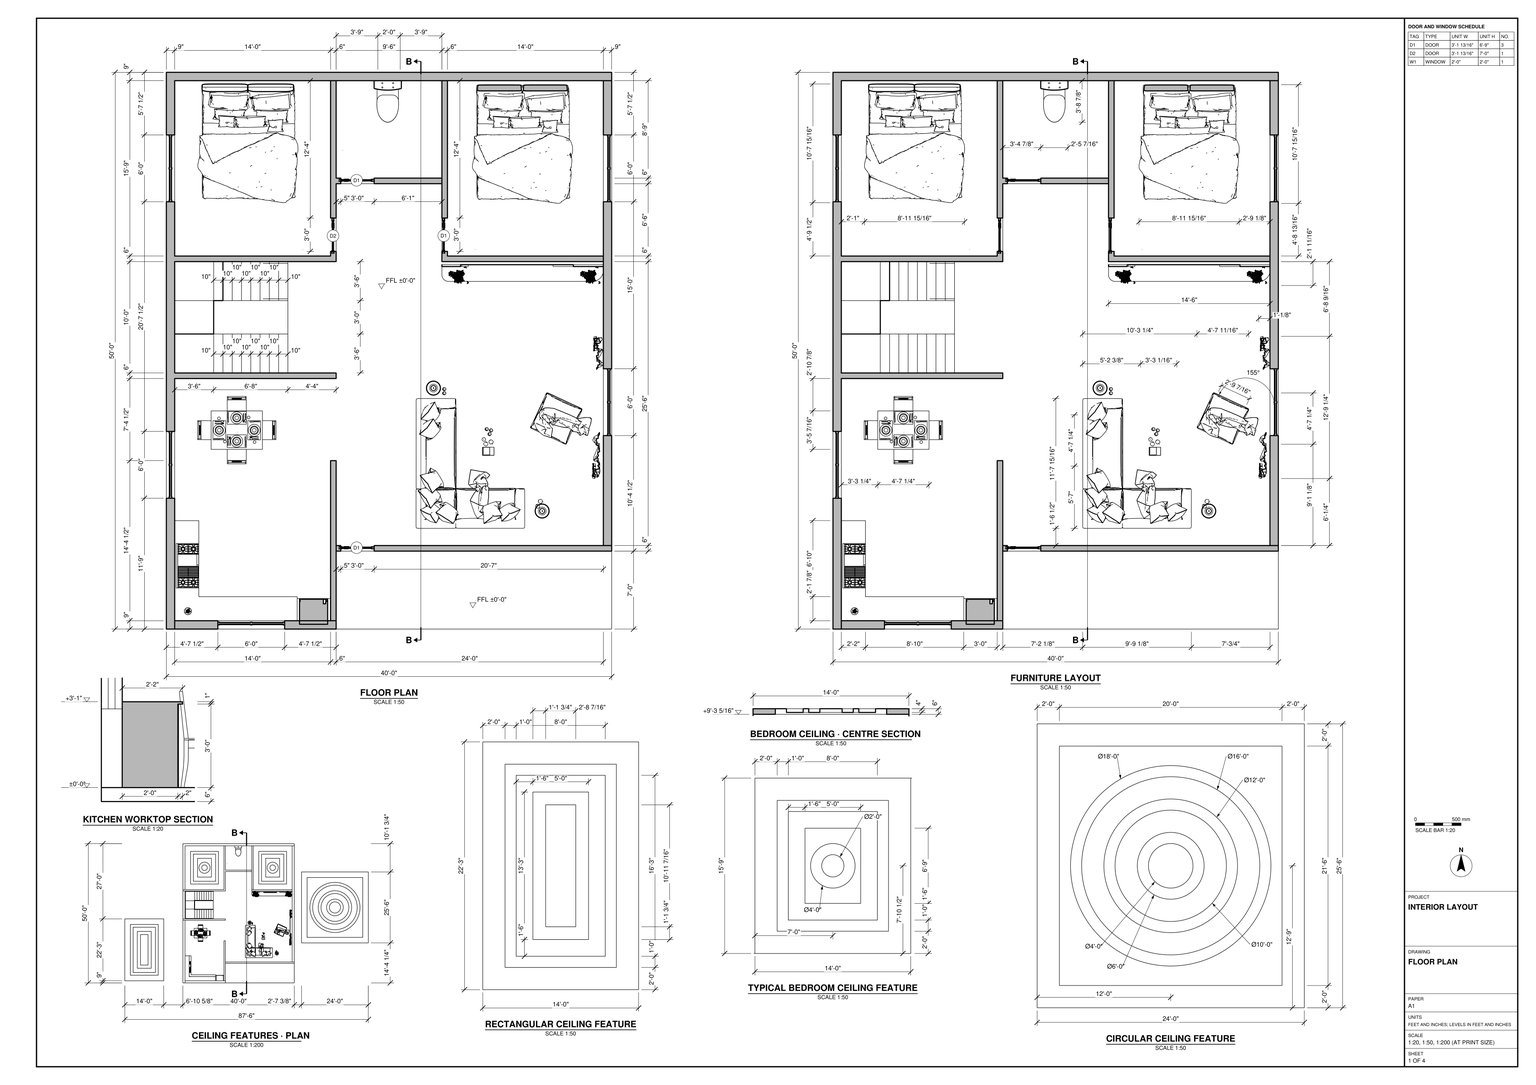
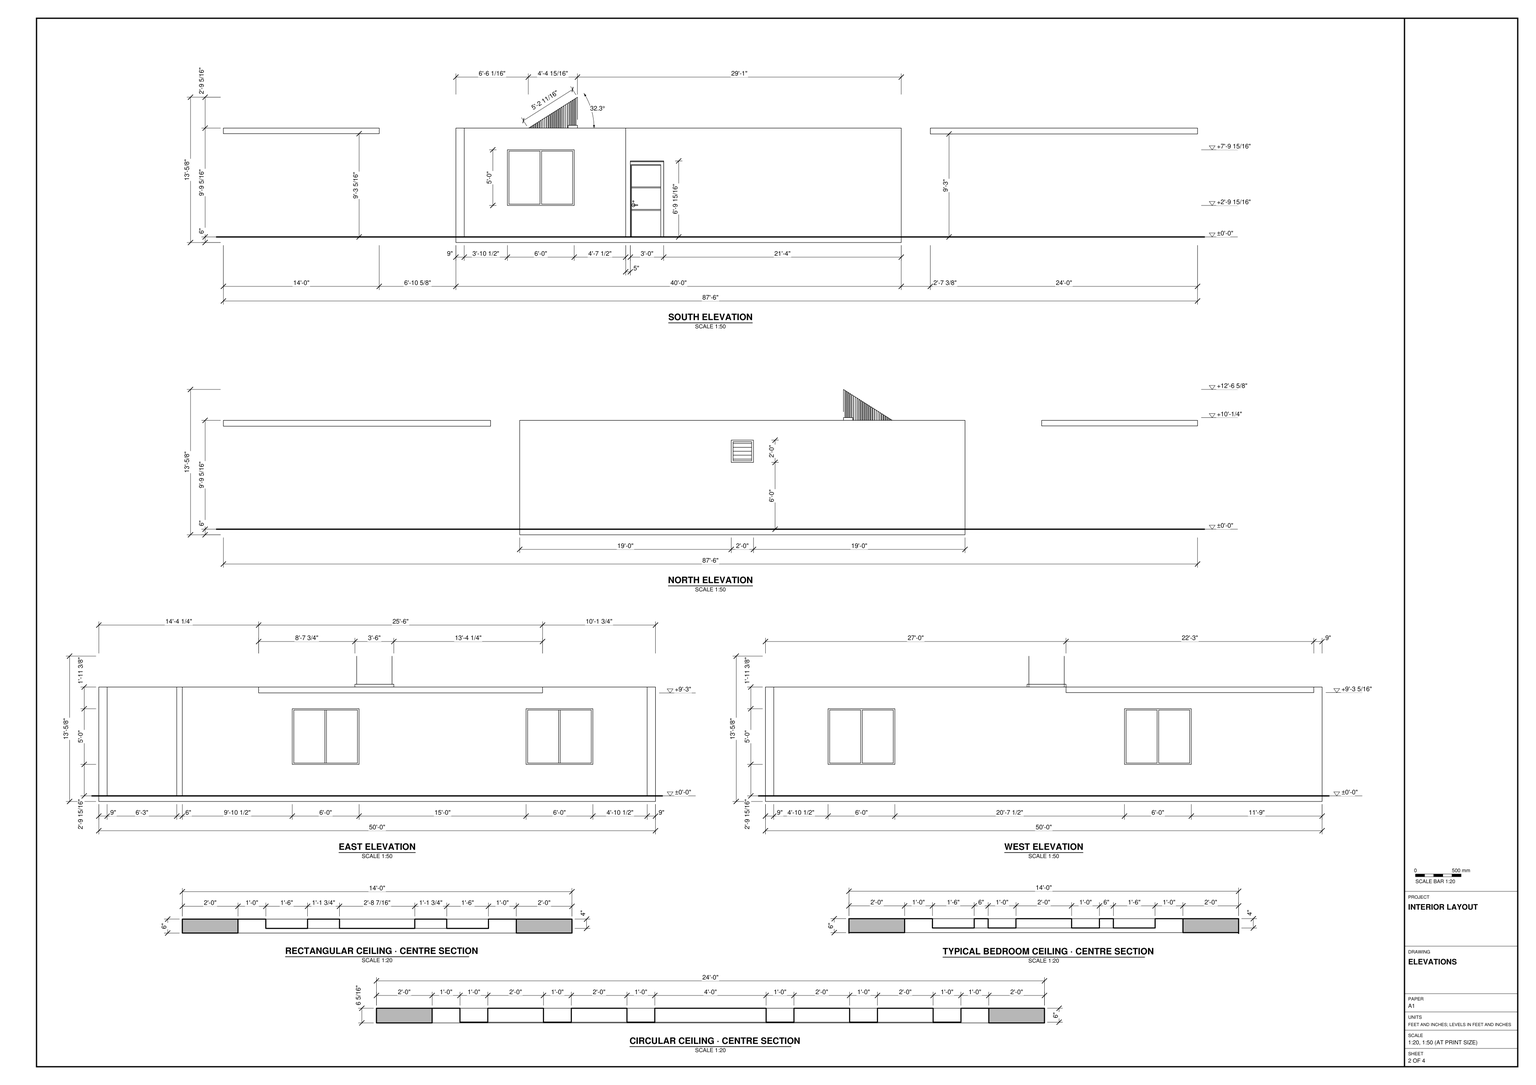
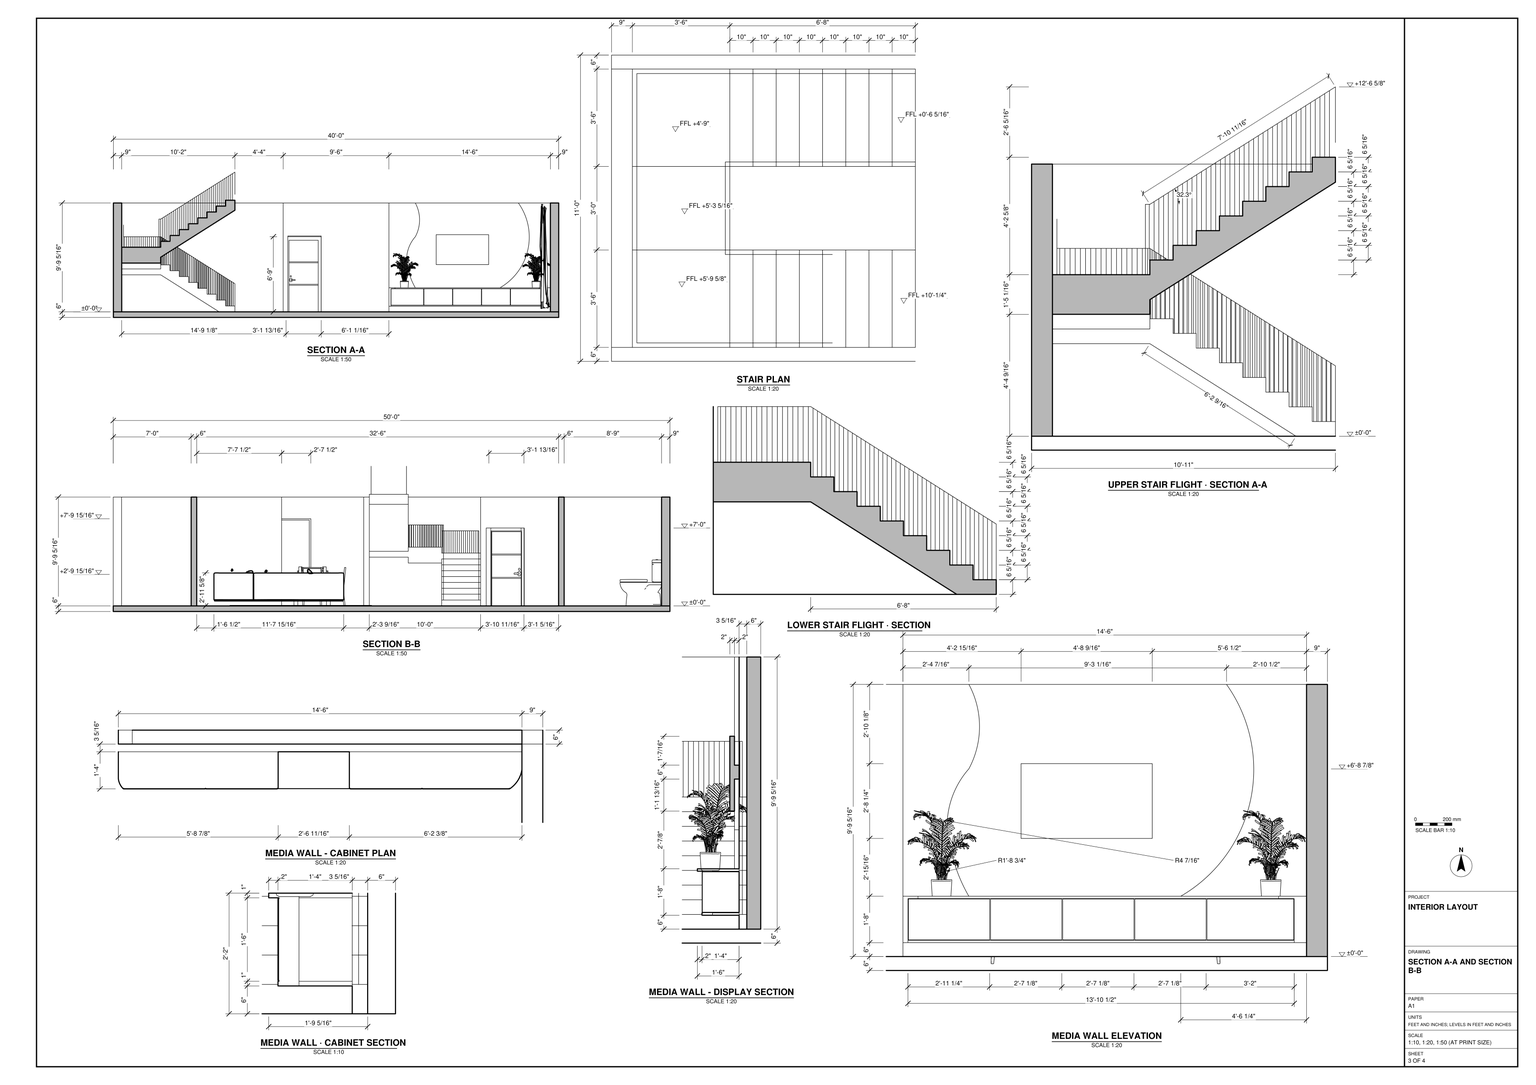
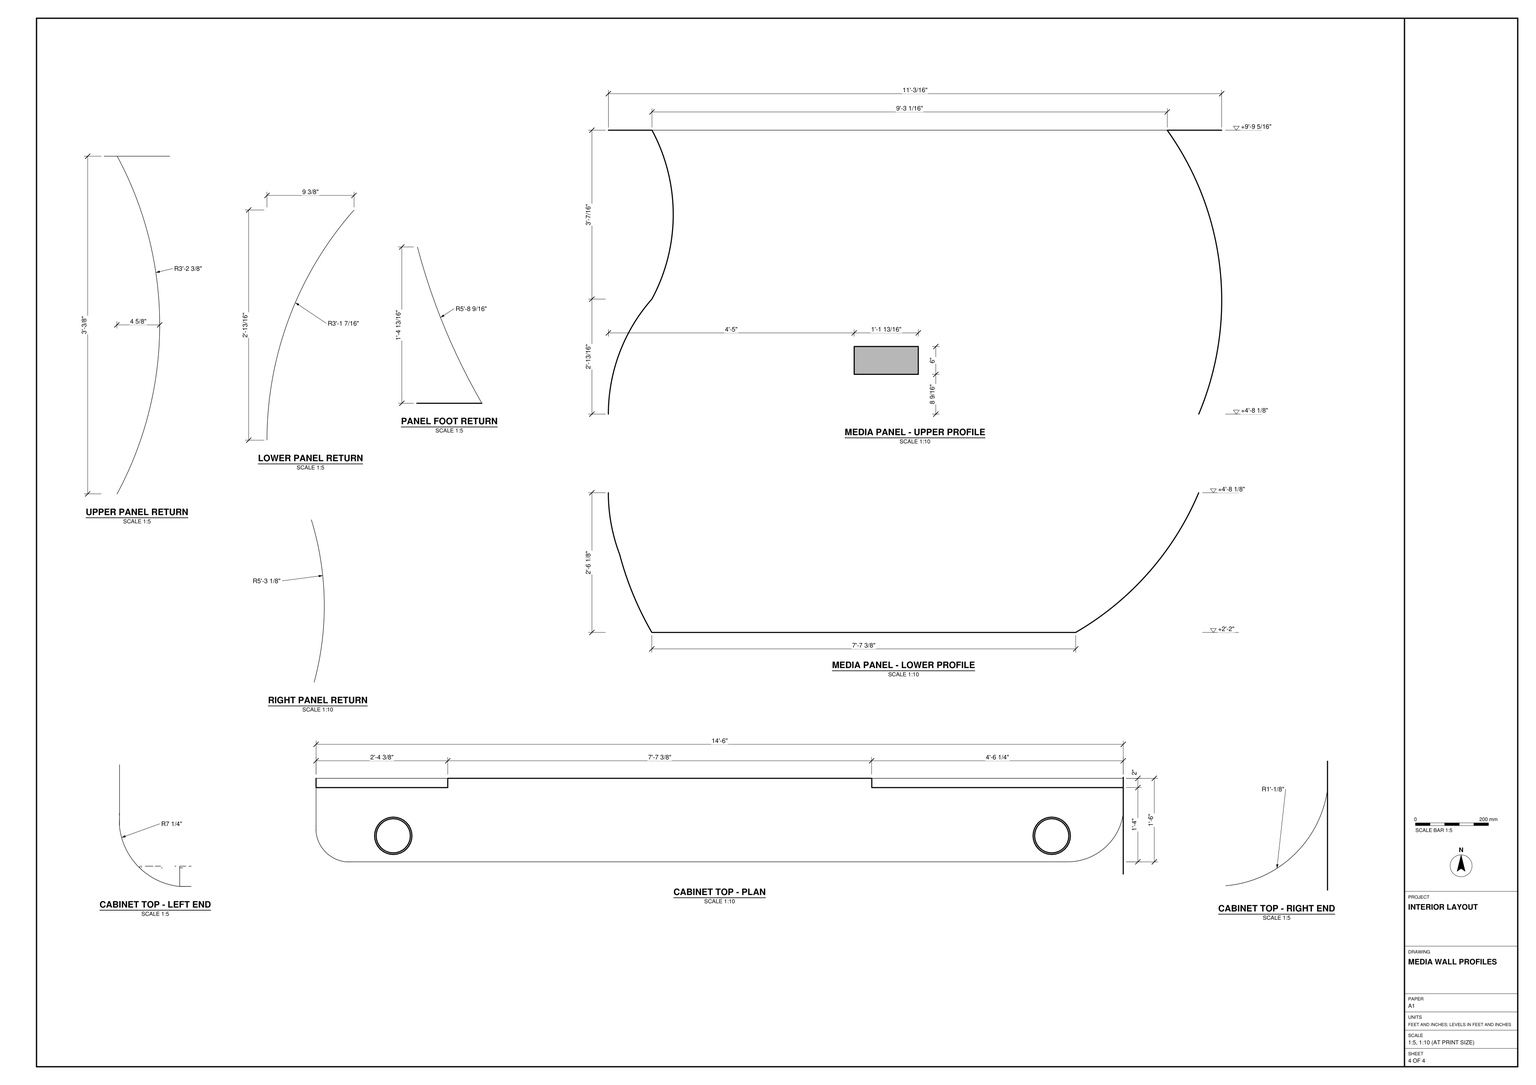
Build the interior in SketchUp from task_files/diagram_01.pdf, working in feet and inches. Set the finished floor at ±0'-0". The complete layout, including the ceiling panels displayed beside the interior, measures 87'-6" along the x-axis, 50'-0" along the y-axis and 10'-6 1/4" in height. The dwelling itself is 40'-0" wide; do not stretch its floor plan to fill the full display width.

Model the floor slab, the 9" exterior walls and the interior partitions at their drawn thicknesses. Preserve the setback at the living room entrance. Place the two bedrooms across the north end with the toilet room between them, and fit the doors and window openings using the plan and elevations. Build the return stair on the west side with its opposing flights, landing and railings.

Fit the kitchen with its L-shaped worktop and base units. Place the dining table and chairs between the kitchen and stair. Arrange the beds, sectional sofa and armchair as shown in the furniture layout. Use the sections to build the low cabinet and curved backing of the media wall opposite the sofa. Model the stepped bedroom ceilings in place and the separate rectangular and circular ceiling features in the positions shown on the ceiling plan. Decor and loose items, including plants and appliances, may be any suitable library components.

Keep shell elements and individual furniture and joinery pieces in separate groups or components, and use components for repeated parts. Save one SketchUp model as output_files/furnished_two_bedroom_interior_with_stepped_ceiling.skp.

# SketchUp Ruby script. Lengths in inches.
U = 1.inch
M = Sketchup.active_model
def pt(a) = Geom::Point3d.new(a.map { |v| v * U })
def face(e, loops, mat)
  f = e.add_face(loops[0].map { |a| pt(a) })
  loops[1..].each { |l| e.add_face(l.map { |a| pt(a) }).erase! }
  f.material = f.back_material = mat if mat
  f
end
# faces: each face lists its corners as indices into pts; further lists are holes
def faces(e, pts, list, mat = nil) = list.each { |f| face(e, (f[0].is_a?(Array) ? f : [f]).map { |l| l.map { |i| pts[i] } }, mat) }
# xy, xz, yz: faces in a plane at the given z, y or x. An outline is a flat list of corners, or four numbers for a rectangle; further outlines are holes
def ring(l) = l.size == 4 ? [[l[0], l[1]], [l[2], l[1]], [l[2], l[3]], [l[0], l[3]]] : l.each_slice(2).to_a
def flat(e, list, mat, &to3) = list.each { |f| face(e, (f[0].is_a?(Array) ? f : [f]).map { |l| ring(l).map { |u, v| to3.(u, v) } }, mat) }
def xy(e, z, list, mat = nil) = flat(e, list, mat) { |x, y| [x, y, z] }
def xz(e, y, list, mat = nil) = flat(e, list, mat) { |x, z| [x, y, z] }
def yz(e, x, list, mat = nil) = flat(e, list, mat) { |y, z| [x, y, z] }
def lines(e, pts, list) = list.each { |a, b| e.add_line(pt(pts[a]), pt(pts[b])) }
# prism: a flat outline (further loops are holes) pulled along v
def prism(e, loops, v, mat = nil)
  f = face(e, loops, mat); d = Geom::Vector3d.new(v.map { |x| x * U })
  f.pushpull(f.normal.samedirection?(d) ? d.length : -d.length)
end
def box(e, o, s, mat = nil) = prism(e, [[o, [o[0] + s[0], o[1], o[2]], [o[0] + s[0], o[1] + s[1], o[2]], [o[0], o[1] + s[1], o[2]]]], [0, 0, s[2]], mat)
def at(x, y, z, deg = 0) = Geom::Transformation.translation(pt([x, y, z])) * Geom::Transformation.rotation(ORIGIN, Z_AXIS, deg.degrees)
def axes(o, x, y, z) = Geom::Transformation.new([*x, 0, *y, 0, *z, 0, *pt(o).to_a, 1])
def part(name) = M.definitions.add(name)
# library, detail: a bought-in or finely detailed component or shape, given as its bounding box
def library(name, o, s) = part(name).tap { |d| box(d.entities, o, s) }
def detail(e, o, s) = box(e.add_group.entities, o, s)
def put(e, d, t, mat = nil) = e.add_instance(d, t).tap { |i| i.material = mat if mat }
def group(e, t, mat = nil) = e.add_group.tap { |g| g.transformation = t; g.material = mat if mat }.entities
root = M.entities
M.materials.add("[Color_008]").color = [30, 30, 30]
M.materials.add("[Color_009]").color = [0, 0, 0]
M.materials.add("[Translucent Glass Gray]").color = [128, 128, 128]
M.materials.add("[Translucent Glass Tinted]1").color = [7, 201, 240]
M.materials.add("[Translucent_Glass_Gray]").color = [128, 128, 128]
M.materials.add("[Wood Cherry Original]").color = [152, 86, 42]
M.materials.add("[Wood Floor Parquet]").color = [145, 89, 39]
c1 = library("A$C150B42AD",[-2.96,-4.03,0],[5.92,8.06,0.01])
c2 = library("main+door",[0,-0.79,0],[47.24,7.88,82.68])
c3 = library("Gas range top",[0,0,34.52],[24.41,48.07,2.63])
c4 = part("Inclined chimney")
g1 = group(c4.entities,at(1.97,2.08,2.89))
xy(g1,0,[[0,7.9,31.3,13.68]])
xy(g1,11.29,[[0,0,31.3,13.68]])
xz(g1,13.68,[[0,0,31.3,11.29]])
yz(g1,0,[[7.9,0,0,11.29,13.68,11.29,13.68,0]])
yz(g1,31.3,[[7.9,0,13.68,0,13.68,11.29,0,11.29]])
g2 = group(c4.entities,at(0,9.85,0.4))
g3 = group(g2,at(0,0.61,0.43))
prism(g3,[[[35.24,0,0],[35.24,-3.39,4.84],[35.24,-3.58,4.7],[35.24,-0.29,0]]],[-35.24,0,0])
g4 = group(g2,at(0,-3.21,4.99))
prism(g4,[[[35.24,-0.2,-0.12],[35.24,-3.16,5],[0,-3.16,5],[0,-0.2,-0.12]]],[0,0.2,0.12])
g5 = group(g2,at(0,-6.27,10.27))
prism(g5,[[[35.24,-0.19,-0.14],[35.24,-3.58,4.7],[0,-3.58,4.7],[0,-0.19,-0.14]]],[0,0.19,0.14])
g6 = group(g2,at(0,0.61,0.43))
prism(g6,[[[35.24,0,0],[35.24,0.96,0],[35.24,-9.52,14.96],[35.24,-10.16,14.51]]],[-35.24,0,0])
g7 = group(c4.entities,at(10.24,3.95,20.8))
box(g7,[0,0,-6.62],[14.76,11.8125,20.56])
g8 = group(c4.entities,at(0,10.1,0))
prism(g8,[[[35.24,0.46,0],[35.24,1.33,0],[35.24,1.33,0.83],[35.24,1.01,0.83],[35.24,0.37,0.83],[35.24,0,0.83],[35.24,0,0.64]]],[-35.24,0,0])
c5 = part("Inclined+chimney")
put(c5.entities,c4,at(34.17,38.97,0.69))
c6 = library("SKT_Nearly Natural 5' Kentia Palm Silk Tree",[-23.18,-17.61,0],[47.48,43.95,59.125])
c7 = library("Component\#33",[0,0,0],[60.64,55.48,158.625])
c8 = library("DINING+TABLE_4+SEATER_+1200mm+x+900mm",[14.07,13.24,0],[72.26,62.1,36.02])
c9 = library("sofa+(2)",[-100.93,-81.02,-0.06],[174.43,145.32,46.54])
c10 = library("Curtain set",[2.63,-1.46,0.02],[153.32,14.02,114.15])
c11 = library("bed",[-25.65,-58.99,0],[75.48,89.46,37.24])
c12 = library("CS300DRT",[0,0,0],[27.18,17.85,30.31])
c13 = library("Group\#13",[0,-2.07,0],[175.11,29.89,117.3125])
c14 = part("ventilator")
g9 = group(c14.entities,at(0,0,0))
xy(g9,0,[[0,0,24,1],[0,1,24,6.83]],"[Wood Floor Parquet]")
xy(g9,1.75,[[2,0,22,6.83]],"[Wood Floor Parquet]")
xy(g9,21.87,[[2,0,22,6.83]],"[Wood Cherry Original]")
xy(g9,23.62,[[0,0,24,1],[0,1,24,6.83]],"[Wood Floor Parquet]")
xz(g9,0,[[[0,0,24,23.62],[2,1.75,22,21.87]]],"[Wood Floor Parquet]")
xz(g9,6.83,[[[0,0,24,23.62],[2,1.75,22,21.87]]],"[Wood Cherry Original]")
yz(g9,0,[[0,0,1,23.62],[1,0,6.83,23.62]],"[Wood Floor Parquet]")
yz(g9,2,[[0,1.75,6.83,1.75,6.83,7.66,0,3.5],[0,3.5,6.83,7.66,6.83,11.8125,0,7.66],[0,7.66,6.83,11.8125,6.83,15.97,0,11.8125],[0,11.8125,6.83,15.97,6.83,20.12,0,15.97],[0,15.97,6.83,20.12,6.83,21.87,0,21.87]],"[Wood Floor Parquet]")
yz(g9,22,[[0,1.75,0,3.5,6.83,7.66,6.83,1.75],[0,3.5,0,7.66,6.83,11.8125,6.83,7.66],[0,7.66,0,11.8125,6.83,15.97,6.83,11.8125],[0,11.8125,0,15.97,6.83,20.12,6.83,15.97],[0,15.97,0,21.87,6.83,21.87,6.83,20.12]],"[Wood Floor Parquet]")
yz(g9,24,[[0,0,1,23.62],[1,0,6.83,23.62]],"[Wood Floor Parquet]")
p = [[2,0,3.5],[2,6.83,7.66],[22,6.83,7.66],[22,0,3.5],[2,6.83,11.8125],[2,0,7.66],
  [22,0,7.66],[22,6.83,11.8125],[2,0,11.8125],[2,6.83,15.97],[22,6.83,15.97],[22,0,11.8125],
  [2,6.83,20.12],[2,0,15.97],[22,0,15.97],[22,6.83,20.12]]
faces(g9,p,[[0,1,2,3],[4,5,6,7],[8,9,10,11]],"[Translucent Glass Tinted]1")
faces(g9,p,[[12,13,14,15]],"[Translucent Glass Gray]")
c15 = part("Group\#2")
xy(c15.entities,0,[[0,0,82.68,1.18]],"[Color_009]")
xy(c15.entities,1.97,[[1.97,0.98,40.35,1.18],[42.32,0.98,80.71,1.18]])
xy(c15.entities,1.97,[[1.97,0,40.35,0.3],[42.32,0,80.71,0.3]],"[Color_009]")
xy(c15.entities,80.71,[[1.97,0,40.35,0.3],[42.32,0,80.71,0.3],[1.97,0.3,40.35,0.98],[42.32,0.3,80.71,0.98],[1.97,0.98,40.35,1.18],
  [42.32,0.98,80.71,1.18]])
xy(c15.entities,82.68,[[0,0,82.68,1.18]],"[Color_008]")
xz(c15.entities,0,[[[0,0,82.68,82.68],[1.97,1.97,40.35,80.71],[42.32,1.97,80.71,80.71]]],"[Color_009]")
xz(c15.entities,0.3,[[1.97,1.97,40.35,80.71],[42.32,1.97,80.71,80.71]],"[Translucent_Glass_Gray]")
xz(c15.entities,0.98,[[1.97,1.97,40.35,80.71],[42.32,1.97,80.71,80.71]],"[Translucent_Glass_Gray]")
xz(c15.entities,1.18,[[[0,0,82.68,82.68],[1.97,1.97,80.71,80.71]],[40.35,1.97,42.32,80.71]],"[Color_009]")
yz(c15.entities,0,[[0,0,1.18,82.68]],"[Color_009]")
yz(c15.entities,1.97,[[0.98,1.97,1.18,80.71]])
yz(c15.entities,1.97,[[0,1.97,0.3,80.71]],"[Color_009]")
yz(c15.entities,40.35,[[0,1.97,0.3,80.71],[0.98,1.97,1.18,80.71]],"[Color_009]")
yz(c15.entities,42.32,[[0,1.97,0.3,80.71],[0.98,1.97,1.18,80.71]])
yz(c15.entities,80.71,[[0,1.97,0.3,80.71],[0.98,1.97,1.18,80.71]],"[Color_009]")
yz(c15.entities,82.68,[[0,0,1.18,82.68]],"[Color_009]")
c16 = library("Group\#6",[0,0,0],[122,120,150.6])
c17 = library("Group\#53",[0,0,-6.3125],[288,306,6.3125])
c18 = library("Group\#54",[0,0,-6],[168,189,6])
c19 = library("Group\#57",[0,0,-6],[168,189,6])
xy(root,0,[[259.625,9,283.625,32.9],[259.625,32.9,283.625,104.9]])
xy(root,0.2,[[283.82,32.9,301.42,33.08],[301.82,32.9,319.42,33.08],[319.82,32.9,355.42,33.08],[355.82,32.9,373.42,33.08],[373.82,32.9,391.42,33.08],
  [283.625,33.1,283.8,49.49],[283.625,49.89,283.8,66.28],[283.625,66.68,283.8,80.9],[283.625,80.9,283.8,83.07],[283.625,83.47,283.8,99.85],
  [283.625,100.25,283.8,104.9],[283.625,104.9,283.8,116.64]])
xy(root,11.8,[[319.82,32.9,355.42,33.08]])
xy(root,12.2,[[319.82,32.9,355.42,33.08]])
xy(root,23.8,[[319.82,32.9,355.42,33.08]])
xy(root,24.2,[[319.82,32.9,355.42,33.08]])
xy(root,35.8,[[283.82,32.9,301.42,33.08],[301.82,32.9,319.42,33.08],[319.82,32.9,355.42,33.08],[355.82,32.9,373.42,33.08],[373.82,32.9,391.42,33.08],
  [283.625,33.1,283.8,49.49],[283.625,49.89,283.8,66.28],[283.625,66.68,283.8,83.07],[283.625,83.47,283.8,99.85],[283.625,100.25,283.8,116.64]])
xy(root,93.9375,[[259.625,9,277.625,116.84],[277.625,9,391.625,27]])
xy(root,94.14,[[277.82,27,300.22,27.18],[300.625,27,323.02,27.18],[323.42,27,345.82,27.18],[346.22,27,368.625,27.18],[369.02,27,391.42,27.18],
  [277.625,27.2,277.8,44.77],[277.625,45.17,277.8,62.74],[277.625,63.14,277.8,80.71],[277.625,81.11,277.8,98.67],[277.625,99.07,277.8,116.64]])
xy(root,117.11,[[277.82,27,300.22,27.18],[300.625,27,323.02,27.18],[323.42,27,345.82,27.18],[346.22,27,368.625,27.18],[369.02,27,391.42,27.18],
  [277.625,27.2,277.8,44.77],[277.625,45.17,277.8,62.74],[277.625,63.14,277.8,80.71],[277.625,81.11,277.8,98.67],[277.625,99.07,277.8,116.64]])
xy(root,117.3125,[[259.625,9,391.625,9,391.625,27,277.625,27,277.625,116.84,259.625,116.84]])
xz(root,9,[[259.625,93.9375,391.625,117.3125]])
xz(root,27,[[[277.625,93.9375,300.42,117.3125],[277.82,94.14,300.22,117.11]],[[300.42,93.9375,323.22,117.3125],[300.625,94.14,323.02,117.11]],[[323.22,93.9375,346.02,117.3125],[323.42,94.14,345.82,117.11]],[[346.02,93.9375,368.82,117.3125],[346.22,94.14,368.625,117.11]],[[368.82,93.9375,391.625,117.3125],[369.02,94.14,391.42,117.11]]])
xz(root,27.18,[[277.82,94.14,300.22,117.11],[300.625,94.14,323.02,117.11],[323.42,94.14,345.82,117.11],[346.22,94.14,368.625,117.11],[369.02,94.14,391.42,117.11]])
xz(root,27.2,[[277.625,94.14,277.8,117.11]])
xz(root,32.9,[[[283.625,0,301.625,36],[283.82,0.2,301.42,35.8]],[[301.625,0,319.625,36],[301.82,0.2,319.42,35.8]],[[319.625,0,355.625,12],[319.82,0.2,355.42,11.8]],[[355.625,0,373.625,36],[355.82,0.2,373.42,35.8]],[[373.625,0,391.625,36],[373.82,0.2,391.42,35.8]],
  [[319.625,12,355.625,24],[319.82,12.2,355.42,23.8]],[[319.625,24,355.625,36],[319.82,24.2,355.42,35.8]]])
xz(root,33.08,[[283.82,0.2,301.42,35.8],[301.82,0.2,319.42,35.8],[319.82,0.2,355.42,11.8],[355.82,0.2,373.42,35.8],[373.82,0.2,391.42,35.8],
  [319.82,12.2,355.42,23.8],[319.82,24.2,355.42,35.8]])
xz(root,33.1,[[283.625,0.2,283.8,35.8]])
xz(root,44.77,[[277.625,94.14,277.8,117.11]])
xz(root,45.17,[[277.625,94.14,277.8,117.11]])
xz(root,49.49,[[283.625,0.2,283.8,35.8]])
xz(root,49.89,[[283.625,0.2,283.8,35.8]])
xz(root,62.74,[[277.625,94.14,277.8,117.11]])
xz(root,63.14,[[277.625,94.14,277.8,117.11]])
xz(root,66.28,[[283.625,0.2,283.8,35.8]])
xz(root,66.68,[[283.625,0.2,283.8,35.8]])
xz(root,80.71,[[277.625,94.14,277.8,117.11]])
xz(root,81.11,[[277.625,94.14,277.8,117.11]])
xz(root,83.07,[[283.625,0.2,283.8,35.8]])
xz(root,83.47,[[283.625,0.2,283.8,35.8]])
xz(root,98.67,[[277.625,94.14,277.8,117.11]])
xz(root,99.07,[[277.625,94.14,277.8,117.11]])
xz(root,99.85,[[283.625,0.2,283.8,35.8]])
xz(root,100.25,[[283.625,0.2,283.8,35.8]])
xz(root,116.64,[[283.625,0.2,283.8,35.8],[277.625,94.14,277.8,117.11]])
xz(root,116.84,[[259.625,93.9375,277.625,117.3125]])
yz(root,259.625,[[9,93.9375,116.84,117.3125]])
yz(root,277.625,[[[27,93.9375,44.97,117.3125],[27.2,94.14,44.77,117.11]],[[44.97,93.9375,62.9375,117.3125],[45.17,94.14,62.74,117.11]],[[62.9375,93.9375,80.91,117.3125],[63.14,94.14,80.71,117.11]],[[80.91,93.9375,98.875,117.3125],[81.11,94.14,98.67,117.11]],[[98.875,93.9375,116.84,117.3125],[99.07,94.14,116.64,117.11]]])
yz(root,277.8,[[27.2,94.14,44.77,117.11],[45.17,94.14,62.74,117.11],[63.14,94.14,80.71,117.11],[81.11,94.14,98.67,117.11],[99.07,94.14,116.64,117.11]])
yz(root,277.82,[[27,94.14,27.18,117.11]])
yz(root,283.625,[[[32.9,0,116.84,36],[66.68,0.2,83.07,35.8],[49.89,0.2,66.28,35.8],[33.1,0.2,49.49,35.8],[83.47,0.2,99.85,35.8],[100.25,0.2,116.64,35.8]]])
yz(root,283.8,[[33.1,0.2,49.49,35.8],[49.89,0.2,66.28,35.8],[66.68,0.2,83.07,35.8],[83.47,0.2,99.85,35.8],[100.25,0.2,116.64,35.8]])
yz(root,283.82,[[32.9,0.2,33.08,35.8]])
yz(root,300.22,[[27,94.14,27.18,117.11]])
yz(root,300.625,[[27,94.14,27.18,117.11]])
yz(root,301.42,[[32.9,0.2,33.08,35.8]])
yz(root,301.82,[[32.9,0.2,33.08,35.8]])
yz(root,319.42,[[32.9,0.2,33.08,12],[32.9,12,33.08,24],[32.9,24,33.08,35.8]])
yz(root,319.82,[[32.9,0.2,33.08,11.8],[32.9,12.2,33.08,23.8],[32.9,24.2,33.08,35.8]])
yz(root,323.02,[[27,94.14,27.18,117.11]])
yz(root,323.42,[[27,94.14,27.18,117.11]])
yz(root,345.82,[[27,94.14,27.18,117.11]])
yz(root,346.22,[[27,94.14,27.18,117.11]])
yz(root,355.42,[[32.9,0.2,33.08,11.8],[32.9,12.2,33.08,23.8],[32.9,24.2,33.08,35.8]])
yz(root,355.82,[[32.9,0.2,33.08,12],[32.9,12,33.08,24],[32.9,24,33.08,35.8]])
yz(root,368.625,[[27,94.14,27.18,117.11]])
yz(root,369.02,[[27,94.14,27.18,117.11]])
yz(root,373.42,[[32.9,0.2,33.08,35.8]])
yz(root,373.82,[[32.9,0.2,33.08,35.8]])
yz(root,391.42,[[32.9,0.2,33.08,35.8],[27,94.14,27.18,117.11]])
yz(root,391.625,[[9,93.9375,27,117.3125]])
# 513 loose lines left out
put(root,c1,axes([490.28,570.1875,0],[4.26064,0,0],[0,4.26064,0],[0,0,4.26064]))
put(root,c2,axes([436.76,482.54,0],[0.8,0,0],[0,0.36,0],[0,0,0.9798]))
put(root,c1,axes([1166.18,532.05,0],[4.26064,0,0],[0,4.26064,0],[0,0,4.26064]))
put(root,c3,at(261.21,44.23,2.48))
put(root,c5,at(314.36,19.5625,59.34,90))
put(root,c6,axes([273.85,19.21,37],[0.59,0,0],[0,0.59,0],[0,0,0.59]))
put(root,c7,axes([424.49,32.9,0],[-0.5,0,0],[0,-0.5,0],[0,0,0.5]))
put(root,c8,axes([267.78,162.56,0],[1.17,0,0],[0,1.17,0],[0,0,1.17]))
put(root,c9,axes([594.47,183.76,0.07],[-1.17,0,0],[0,-1.17,0],[0,0,1.17]))
put(root,c10,at(709.07,318.15,3.14,-90))
put(root,c11,axes([321.28,543.86,0],[1.43,0,0],[0,1.43,0],[0,0,1.43]))
put(root,c11,axes([617.21,543.15,-3.12],[1.43,0,0],[0,1.43,0],[0,0,1.43]))
put(root,c12,axes([474.5,591,0],[0,-1.65,0],[1.65,0,0],[0,0,1.65]))
g10 = group(root,at(250.625,0,-6))
xy(g10,0,[[0,0,480,600]])
xy(g10,6,[[[0,0,480,600],[9,9,9,116.84,33,116.84,33,32.9,141,32.9,141,9]]])
xy(g10,42,[[33,32.9,35,116.84],[35,32.9,141,34.9]])
xy(g10,43,[[9,9,141,9,141,34.9,35,34.9,35,116.84,9,116.84]])
xz(g10,0,[[0,0,480,6]])
xz(g10,9,[[9,6,141,43]])
xz(g10,32.9,[[33,6,141,42]])
xz(g10,34.9,[[35,42,141,43]])
xz(g10,116.84,[[9,6,9,43,35,43,35,42,33,42,33,6]])
xz(g10,600,[[0,0,480,6]])
yz(g10,0,[[0,0,600,6]])
yz(g10,9,[[9,6,116.84,43]])
yz(g10,33,[[32.9,6,116.84,42]])
yz(g10,35,[[34.9,42,116.84,43]])
yz(g10,141,[[9,6,32.9,6,32.9,42,34.9,42,34.9,43,9,43]])
yz(g10,480,[[0,0,600,6]])
put(root,c13,at(547.6,370.3,0))
g11 = group(root,at(250.625,0,0))
xy(g11,0,[[0,0,9,141],[9,0,55.5,9],[55.5,0,183,9],[177,9,183,181.5],[183,84,188,90],
  [224,84,480,90],[471,90,480,208.5],[0,141,9,270],[471,208.5,480,460.5],[297,396,471,402],
  [0,402,9,460.5],[297,402,303,407],[177,443,183,591],[297,443,303,591],[0,460.5,9,591],
  [471,460.5,480,591],[183,480,188,486],[224,480,297,486],[0,591,228,600],[228,591,480,600]])
xy(g11,33.9375,[[55.5,0,127.5,9],[0,141,9,213],[471,208.5,480,280.5],[0,460.5,9,532.5],[471,460.5,480,532.5]])
xy(g11,72,[[228,591,252,600]])
xy(g11,81.75,[[188,480,224,486]])
xy(g11,81.9375,[[188,84,224,90]])
xy(g11,84,[[177,407,183,443],[297,407,303,443]])
xy(g11,93.9375,[[55.5,0,127.5,9],[0,141,9,213],[471,208.5,480,280.5],[0,460.5,9,532.5],[471,460.5,480,532.5]])
xy(g11,96,[[228,591,252,600]])
xy(g11,117.3125,[[0,0,9,270],[9,0,183,9],[177,9,183,181.5],[183,84,480,90],[471,90,480,591],
  [0,270,183,276],[0,276,9,396],[0,396,183,396,183,480,297,480,297,486,183,486,183,591,177,591,177,402,0,402],[297,396,471,402],[0,402,9,402,9,591,480,591,480,600,0,600],
  [297,402,303,591]])
xz(g11,0,[[0,0,9,117.3125],[[9,0,183,117.3125],[55.5,33.9375,127.5,93.9375]]])
xz(g11,9,[[[9,0,177,117.3125],[55.5,33.9375,127.5,93.9375]],[177,0,183,117.3125]])
xz(g11,84,[[183,0,188,0,188,81.9375,224,81.9375,224,0,480,0,480,117.3125,183,117.3125]])
xz(g11,90,[[183,0,183,117.3125,471,117.3125,471,0,224,0,224,81.9375,188,81.9375,188,0],[471,0,480,117.3125]])
xz(g11,141,[[0,33.9375,9,93.9375]])
xz(g11,181.5,[[177,0,183,117.3125]])
xz(g11,208.5,[[471,33.9375,480,93.9375]])
xz(g11,213,[[0,33.9375,9,93.9375]])
xz(g11,270,[[9,0,183,117.3125]])
xz(g11,276,[[9,0,183,117.3125]])
xz(g11,280.5,[[471,33.9375,480,93.9375]])
xz(g11,396,[[9,0,183,117.3125],[297,0,471,117.3125]])
xz(g11,402,[[9,0,177,117.3125],[303,0,471,117.3125]])
xz(g11,407,[[177,0,183,84],[297,0,303,84]])
xz(g11,443,[[177,0,183,84],[297,0,303,84]])
xz(g11,460.5,[[0,33.9375,9,93.9375],[471,33.9375,480,93.9375]])
xz(g11,480,[[183,0,188,0,188,81.75,224,81.75,224,0,297,0,297,117.3125,183,117.3125]])
xz(g11,486,[[183,0,183,117.3125,297,117.3125,297,0,224,0,224,81.75,188,81.75,188,0]])
xz(g11,532.5,[[0,33.9375,9,93.9375],[471,33.9375,480,93.9375]])
xz(g11,591,[[9,0,177,117.3125],[177,0,183,117.3125],[[183,0,297,117.3125],[228,72,252,96]],[297,0,303,117.3125],[303,0,471,117.3125],
  [471,0,480,117.3125]])
xz(g11,600,[[[0,0,480,117.3125],[228,72,252,96]]])
yz(g11,0,[[[0,0,591,117.3125],[460.5,33.9375,532.5,93.9375],[141,33.9375,213,93.9375]],[591,0,600,117.3125]])
yz(g11,9,[[0,0,9,117.3125],[[9,0,270,117.3125],[141,33.9375,213,93.9375]],[276,0,396,117.3125],[[402,0,591,117.3125],[460.5,33.9375,532.5,93.9375]]])
yz(g11,55.5,[[0,33.9375,9,93.9375]])
yz(g11,127.5,[[0,33.9375,9,93.9375]])
yz(g11,177,[[9,0,181.5,117.3125],[402,0,402,117.3125,591,117.3125,591,0,443,0,443,84,407,84,407,0]])
yz(g11,183,[[0,0,9,117.3125],[9,0,84,117.3125],[84,0,90,117.3125],[90,0,181.5,117.3125],[270,0,276,117.3125],
  [396,0,402,0,402,84,443,84,443,0,480,0,480,117.3125,396,117.3125],[402,0,407,84],[486,0,591,117.3125]])
yz(g11,188,[[84,0,90,81.9375],[480,0,486,81.75]])
yz(g11,224,[[84,0,90,81.9375],[480,0,486,81.75]])
yz(g11,228,[[591,72,600,96]])
yz(g11,252,[[591,72,600,96]])
yz(g11,297,[[396,0,396,117.3125,480,117.3125,480,0,443,0,443,84,407,84,407,0],[480,0,486,117.3125],[486,0,591,117.3125]])
yz(g11,303,[[402,0,407,0,407,84,443,84,443,0,591,0,591,117.3125,402,117.3125]])
yz(g11,471,[[[90,0,396,117.3125],[208.5,33.9375,280.5,93.9375]],[396,0,402,117.3125],[[402,0,591,117.3125],[460.5,33.9375,532.5,93.9375]]])
yz(g11,480,[[84,0,90,117.3125],[[90,0,591,117.3125],[208.5,33.9375,280.5,93.9375],[460.5,33.9375,532.5,93.9375]],[591,0,600,117.3125]])
# 4 loose lines left out
put(g11,c2,axes([186.13,86.54,0],[0.8,0,0],[0,0.36,0],[0,0,0.9798]))
put(g11,c14,axes([228,591,72],[1,0,0],[0,1,0],[0,0,1.016]))
put(g11,c2,axes([178.49,442.72,0],[0,-0.8,0],[0.36,0,0],[0,0,1.016]))
put(g11,c2,axes([297.84,442.82,0],[0,-0.8,0],[0.36,0,0],[0,0,0.9798]))
put(g11,c15,axes([2.95,532.5,33.9375],[0,-0.87086,0],[2.5,0,0],[0,0,0.72571]))
put(g11,c15,axes([2.95,213,33.9375],[0,-0.87086,0],[2.5,0,0],[0,0,0.72571]))
put(g11,c15,axes([475.5,280.5,33.9375],[0,-0.87086,0],[2.5,0,0],[0,0,0.72571]))
put(g11,c15,axes([475.5,532.5,33.9375],[0,-0.87086,0],[2.5,0,0],[0,0,0.72571]))
put(g11,c15,axes([55.5,4.5,33.9375],[0.87086,0,0],[0,2.5,0],[0,0,0.72571]))
put(root,c16,at(259.625,276,0))
put(root,c17,at(761.98,172.26,117.3125))
put(root,c18,at(553.625,402,117.3125))
put(root,c19,at(259.625,402,117.3125))
g12 = group(root,at(0,9,117.3125))
xy(g12,-6,[[[0,0,168,267],[24,24,144,243]]])
xy(g12,-4,[[[36,36,132,231],[54,54,114,213]],[67.77,67.77,100.23,199.23]])
xy(g12,0,[[[0,0,168,267],[24,24,144,243]],[[24,24,144,243],[36,36,132,231]],[[54,54,114,213],[67.77,67.77,100.23,199.23]]])
xz(g12,0,[[0,-6,168,0]])
xz(g12,24,[[24,-6,144,0]])
xz(g12,36,[[36,-4,132,0]])
xz(g12,54,[[54,-4,114,0]])
xz(g12,67.77,[[67.77,-4,100.23,0]])
xz(g12,199.23,[[67.77,-4,100.23,0]])
xz(g12,213,[[54,-4,114,0]])
xz(g12,231,[[36,-4,132,0]])
xz(g12,243,[[24,-6,144,0]])
xz(g12,267,[[0,-6,168,0]])
yz(g12,0,[[0,-6,267,0]])
yz(g12,24,[[24,-6,243,0]])
yz(g12,36,[[36,-4,231,0]])
yz(g12,54,[[54,-4,213,0]])
yz(g12,67.77,[[67.77,-4,199.23,0]])
yz(g12,100.23,[[67.77,-4,199.23,0]])
yz(g12,114,[[54,-4,213,0]])
yz(g12,132,[[36,-4,231,0]])
yz(g12,144,[[24,-6,243,0]])
yz(g12,168,[[0,-6,267,0]])
